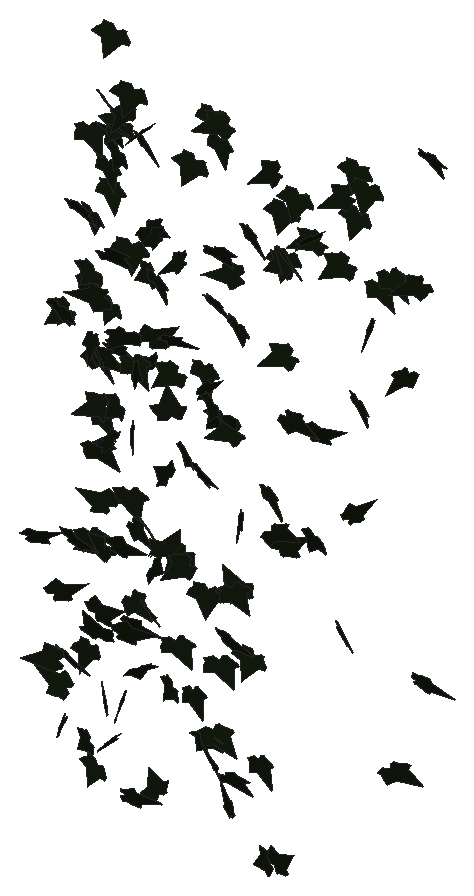
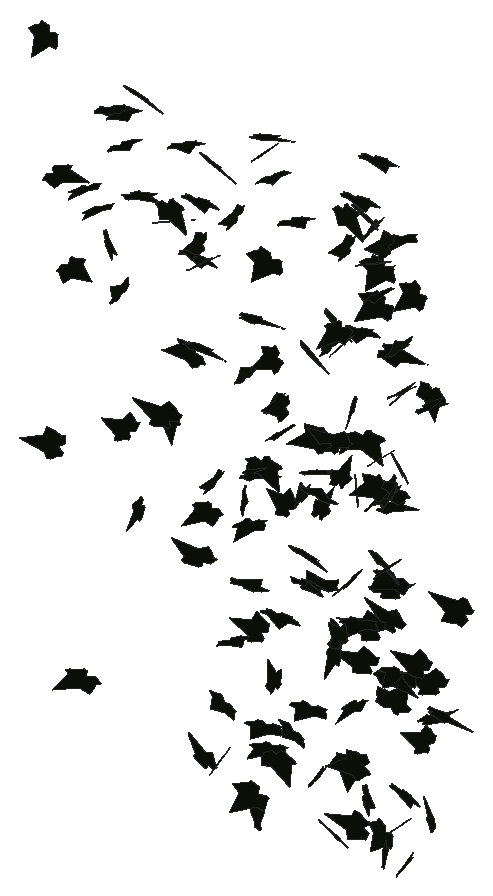
# SketchUp Ruby script. Lengths in inches.
U = 1.inch
M = Sketchup.active_model
def pt(a) = Geom::Point3d.new(a.map { |v| v * U })
def face(e, loops, mat)
  f = e.add_face(loops[0].map { |a| pt(a) })
  loops[1..].each { |l| e.add_face(l.map { |a| pt(a) }).erase! }
  f.material = f.back_material = mat if mat
  f
end
# faces: each face lists its corners as indices into pts; further lists are holes
def faces(e, pts, list, mat = nil) = list.each { |f| face(e, (f[0].is_a?(Array) ? f : [f]).map { |l| l.map { |i| pts[i] } }, mat) }
# xy, xz, yz: faces in a plane at the given z, y or x. An outline is a flat list of corners, or four numbers for a rectangle; further outlines are holes
def ring(l) = l.size == 4 ? [[l[0], l[1]], [l[2], l[1]], [l[2], l[3]], [l[0], l[3]]] : l.each_slice(2).to_a
def flat(e, list, mat, &to3) = list.each { |f| face(e, (f[0].is_a?(Array) ? f : [f]).map { |l| ring(l).map { |u, v| to3.(u, v) } }, mat) }
def xy(e, z, list, mat = nil) = flat(e, list, mat) { |x, y| [x, y, z] }
def xz(e, y, list, mat = nil) = flat(e, list, mat) { |x, z| [x, y, z] }
def yz(e, x, list, mat = nil) = flat(e, list, mat) { |y, z| [x, y, z] }
def lines(e, pts, list) = list.each { |a, b| e.add_line(pt(pts[a]), pt(pts[b])) }
# prism: a flat outline (further loops are holes) pulled along v
def prism(e, loops, v, mat = nil)
  f = face(e, loops, mat); d = Geom::Vector3d.new(v.map { |x| x * U })
  f.pushpull(f.normal.samedirection?(d) ? d.length : -d.length)
end
def box(e, o, s, mat = nil) = prism(e, [[o, [o[0] + s[0], o[1], o[2]], [o[0] + s[0], o[1] + s[1], o[2]], [o[0], o[1] + s[1], o[2]]]], [0, 0, s[2]], mat)
def at(x, y, z, deg = 0) = Geom::Transformation.translation(pt([x, y, z])) * Geom::Transformation.rotation(ORIGIN, Z_AXIS, deg.degrees)
def axes(o, x, y, z) = Geom::Transformation.new([*x, 0, *y, 0, *z, 0, *pt(o).to_a, 1])
def part(name) = M.definitions.add(name)
# library, detail: a bought-in or finely detailed component or shape, given as its bounding box
def library(name, o, s) = part(name).tap { |d| box(d.entities, o, s) }
def detail(e, o, s) = box(e.add_group.entities, o, s)
def put(e, d, t, mat = nil) = e.add_instance(d, t).tap { |i| i.material = mat if mat }
def group(e, t, mat = nil) = e.add_group.tap { |g| g.transformation = t; g.material = mat if mat }.entities
root = M.entities
M.materials.add("1026 AP 7946 SUNNY SIDE UP").color = [254, 231, 186]
M.materials.add("efeu1").color = [18, 25, 13]
c1 = part("ivyleaf_9")
p = [[1.54,2.16,1.25],[1.36,2.04,1.19],[-0.21,0.99,0.68],[-0.71,1.11,0.82],[-0.85,0.86,0.67],[-0.8,0.17,0.21],
  [-0.9,-0.01,0.1],[-0.67,-0.16,-0.02],[-0.08,-0.08,-0.05],[-0.03,-0.6,-0.4],[0.65,-0.88,-0.66],[0.83,-0.6,-0.49],
  [1.29,-0.42,-0.43],[1.8125,-0.07,-0.26],[1.21,0.44,0.15]]
faces(c1.entities,p,[[0,1,2,3,4,5,6,7,8,9,10,11,12,13,14]],"efeu1")
put(root,c1,axes([176.66,210.71,296.68],[-0.62079,-0.06048,-0.24475],[0.37867,-0.01488,-0.40905],[0.06932,-0.46036,0.04263]),"1026 AP 7946 SUNNY SIDE UP")
put(root,c1,axes([176.78,208.77,316.86],[-0.34325,-0.29743,0.3129],[-0.25777,-0.25818,-0.38123],[0.61879,-0.27253,0.01475]),"1026 AP 7946 SUNNY SIDE UP")
put(root,c1,axes([176.43,211.22,321.1875],[-0.03798,-0.39245,0.26497],[0.11301,-0.2598,-0.3995],[0.73105,0.01977,0.07552]),"1026 AP 7946 SUNNY SIDE UP")
put(root,c1,axes([176.24,206.52,304.73],[0.51781,0.27509,-0.19939],[0.19907,0.15193,0.44169],[0.49153,-0.35133,0.03117]),"1026 AP 7946 SUNNY SIDE UP")
put(root,c1,axes([176.3,212.23,327.35],[0.50505,-0.33544,0.1326],[0.09947,-0.11973,-0.47773],[0.55722,0.32541,-0.0349]),"1026 AP 7946 SUNNY SIDE UP")
put(root,c1,axes([176.2,209.78,303.16],[0.29433,-0.17747,0.41107],[0.49315,-0.24903,-0.26646],[0.47991,0.36475,0.02171]),"1026 AP 7946 SUNNY SIDE UP")
put(root,c1,axes([176.51,211.81,309.54],[0.19314,-0.42841,-0.13884],[-0.02652,0.13271,-0.45791],[0.70454,0.12244,0.02083]),"1026 AP 7946 SUNNY SIDE UP")
put(root,c1,axes([176.93,208.05,317.375],[0.51444,0.00554,-0.35204],[-0.52619,-0.09112,-0.33208],[-0.10941,0.46425,-0.05816]),"1026 AP 7946 SUNNY SIDE UP")
put(root,c1,axes([176.74,212.39,315.56],[-0.17337,-0.35996,0.21476],[-0.02551,-0.21388,-0.38676],[0.65519,-0.10358,0.04177]),"1026 AP 7946 SUNNY SIDE UP")
put(root,c1,axes([176.875,211.03,313.57],[0.46463,-0.22327,-0.28441],[-0.39252,0.12246,-0.37832],[0.39483,0.38449,-0.04142]),"1026 AP 7946 SUNNY SIDE UP")
put(root,c1,axes([176.66,210.78,303.15],[-0.25406,-0.21807,-0.38632],[0.38165,0.28462,-0.27751],[0.56331,-0.29119,0.01378]),"1026 AP 7946 SUNNY SIDE UP")
put(root,c1,axes([176.79,211.96,325.92],[0.69115,0.13249,-0.08852],[-0.10161,-0.08337,-0.46936],[-0.22728,0.44019,-0.05935]),"1026 AP 7946 SUNNY SIDE UP")
put(root,c1,axes([176.97,210.64,318.3],[-0.35108,-0.28922,0.29586],[-0.041,-0.31837,-0.35105],[0.64141,-0.17866,0.1395]),"1026 AP 7946 SUNNY SIDE UP")
put(root,c1,axes([177.51,210.74,302.82],[0.026,-0.01704,-0.47108],[-0.57664,-0.27401,-0.00474],[-0.43009,0.36634,-0.02212]),"1026 AP 7946 SUNNY SIDE UP")
put(root,c1,axes([176.93,210.64,314.49],[-0.43021,0.02432,-0.39229],[0.56896,-0.1327,-0.27724],[-0.19109,-0.44984,0.05771]),"1026 AP 7946 SUNNY SIDE UP")
put(root,c1,axes([176.74,211.29,313.15],[0.35166,-0.39736,-0.04156],[-0.03147,0.03244,-0.46955],[0.62688,0.22453,-0.00026]),"1026 AP 7946 SUNNY SIDE UP")
put(root,c1,axes([177.28,211.3,293.05],[-0.00904,-0.18472,0.40636],[0.04608,0.39447,0.19255],[-0.68482,0.02898,0.00759]),"1026 AP 7946 SUNNY SIDE UP")
put(root,c1,axes([176.75,211.08,313.36],[0.0638,-0.0925,-0.47457],[0.3914,0.39579,-0.05704],[0.62566,-0.23817,0.08408]),"1026 AP 7946 SUNNY SIDE UP")
put(root,c1,axes([176.99,209.97,318.18],[0.28007,-0.41904,-0.12282],[-0.08877,0.10292,-0.46833],[0.67825,0.1865,-0.01058]),"1026 AP 7946 SUNNY SIDE UP")
put(root,c1,axes([177.09,207.82,293.42],[0.05621,0.26537,0.34627],[-0.06691,-0.3319,0.27391],[0.66819,-0.05556,-0.0017]),"1026 AP 7946 SUNNY SIDE UP")
put(root,c1,axes([177.04,210.25,326.7],[-0.08134,-0.41139,-0.23378],[0.09107,0.21861,-0.42499],[0.73134,-0.07297,0.02692]),"1026 AP 7946 SUNNY SIDE UP")
put(root,c1,axes([177.34,212.43,326.11],[-0.48774,-0.32332,0.1613],[0.00489,-0.21148,-0.43966],[0.56611,-0.27674,0.14276]),"1026 AP 7946 SUNNY SIDE UP")
put(root,c1,axes([177.25,209.93,291.82],[-0.16792,-0.16998,0.40395],[-0.12439,-0.39031,-0.1983],[0.66179,-0.11649,0.06522]),"1026 AP 7946 SUNNY SIDE UP")
put(root,c1,axes([176.87,207.82,301.1],[0.04149,0.01406,0.48813],[0.72236,0.11593,-0.02923],[-0.18327,0.4601,-0.00469]),"1026 AP 7946 SUNNY SIDE UP")
put(root,c1,axes([177.41,211.85,331.65],[-0.62146,-0.24372,-0.12609],[0.20704,0.01545,-0.475],[0.37444,-0.41305,0.05337]),"1026 AP 7946 SUNNY SIDE UP")
put(root,c1,axes([177.02,210.83,308.28],[-0.16999,-0.13214,-0.44594],[0.48022,0.3061,-0.17335],[0.52367,-0.3236,0.01421]),"1026 AP 7946 SUNNY SIDE UP")
put(root,c1,axes([177.11,208.91,322.98],[0.73184,-0.07926,-0.02833],[-0.05326,-0.0385,-0.48454],[0.12044,0.46462,-0.04216]),"1026 AP 7946 SUNNY SIDE UP")
put(root,c1,axes([178.16,206.2,298.44],[-0.59478,0.131,0.26622],[-0.40522,0.03937,-0.41013],[-0.20586,-0.45599,0.03816]),"1026 AP 7946 SUNNY SIDE UP")
put(root,c1,axes([177.15,211.8,313.65],[0.64815,-0.02989,0.13586],[0.1987,-0.06695,-0.42238],[0.07641,0.42763,-0.05406]),"1026 AP 7946 SUNNY SIDE UP")
put(root,c1,axes([178.14,210.6875,308.99],[-0.41016,0.35242,0.08873],[-0.11772,0.049,-0.45031],[-0.55742,-0.26966,0.02981]),"1026 AP 7946 SUNNY SIDE UP")
put(root,c1,axes([178.24,209.89,311.34],[-0.50112,-0.17584,0.30822],[-0.37278,-0.18818,-0.37394],[0.40035,-0.39531,0.03761]),"1026 AP 7946 SUNNY SIDE UP")
put(root,c1,axes([177.4,207.83,297.77],[0.37377,-0.27426,0.31055],[0.33544,-0.21572,-0.37483],[0.54814,0.31903,0.01762]),"1026 AP 7946 SUNNY SIDE UP")
put(root,c1,axes([177.74,210.85,324.68],[0.06205,-0.47249,0.0648],[0.0049,-0.06555,-0.48883],[0.75005,0.03952,-0.00217]),"1026 AP 7946 SUNNY SIDE UP")
put(root,c1,axes([178.03,210.77,323.5],[-0.05815,-0.46712,-0.02027],[-0.00965,0.01756,-0.48257],[0.73493,-0.03673,-0.00794]),"1026 AP 7946 SUNNY SIDE UP")
put(root,c1,axes([178.92,209.31,306.2],[-0.07979,0.08198,0.45897],[-0.70589,-0.06557,-0.04067],[0.0897,-0.44311,0.0882]),"1026 AP 7946 SUNNY SIDE UP")
put(root,c1,axes([178.73,211.21,327.9],[-0.63622,-0.01116,-0.25311],[0.36454,-0.17488,-0.38627],[-0.1288,-0.43985,0.15701]),"1026 AP 7946 SUNNY SIDE UP")
put(root,c1,axes([178.91,210.78,315.37],[0.21758,0.24064,-0.39838],[-0.25627,-0.35276,-0.28729],[-0.6707,0.21285,-0.01946]),"1026 AP 7946 SUNNY SIDE UP")
put(root,c1,axes([178.14,211.87,298.05],[0.56527,0.0027,0.27538],[0.41884,-0.04098,-0.36889],[0.03506,0.44609,-0.03292]),"1026 AP 7946 SUNNY SIDE UP")
put(root,c1,axes([178.49,211.61,305.74],[-0.25565,-0.34144,-0.2904],[0.22633,0.24104,-0.38757],[0.65634,-0.21612,0.02053]),"1026 AP 7946 SUNNY SIDE UP")
put(root,c1,axes([179.12,205.67,297.49],[-0.36991,-0.40501,-0.08415],[-0.06792,-0.06671,0.48211],[-0.6454,0.23916,-0.0025]),"1026 AP 7946 SUNNY SIDE UP")
put(root,c1,axes([178.79,211.52,328.87],[-0.6171,-0.2234,-0.1631],[0.26314,0.02054,-0.46078],[0.33931,-0.42221,0.06072]),"1026 AP 7946 SUNNY SIDE UP")
put(root,c1,axes([178.83,210.3125,311.43],[-0.17688,-0.26822,0.33727],[-0.17166,-0.31053,-0.30116],[0.64489,-0.15622,0.01234]),"1026 AP 7946 SUNNY SIDE UP")
put(root,c1,axes([179.44,208.25,318.75],[-0.25175,-0.10611,-0.45155],[-0.45796,-0.32996,0.19022],[-0.54021,0.32917,0.04918]),"1026 AP 7946 SUNNY SIDE UP")
put(root,c1,axes([179.28,208.19,299.375],[0.44654,-0.11305,0.36897],[-0.48891,0.18251,0.31384],[-0.33295,-0.41961,0.034]),"1026 AP 7946 SUNNY SIDE UP")
put(root,c1,axes([179.13,208.9,292.76],[0.19534,0.3464,0.30483],[0.15127,0.27775,-0.37748],[-0.69813,0.1571,0.0035]),"1026 AP 7946 SUNNY SIDE UP")
put(root,c1,axes([179.14,209.95,326.17],[-0.08365,-0.33255,0.34235],[-0.02163,-0.33509,-0.34771],[0.74102,-0.04732,0.02849]),"1026 AP 7946 SUNNY SIDE UP")
put(root,c1,axes([179.04,211.83,326.15],[0.4373,-0.3765,0.06903],[0.02872,-0.07231,-0.48177],[0.60122,0.2773,-0.02719]),"1026 AP 7946 SUNNY SIDE UP")
put(root,c1,axes([179.54,211.82,313.14],[0.14933,0.15978,0.43145],[-0.45831,-0.30202,0.18543],[0.53373,-0.30405,0.03852]),"1026 AP 7946 SUNNY SIDE UP")
put(root,c1,axes([179.44,210.01,295.16],[-0.30628,0.09838,-0.43053],[0.51909,-0.26004,-0.2228],[-0.43296,-0.38137,0.03744]),"1026 AP 7946 SUNNY SIDE UP")
put(root,c1,axes([179.53,207.67,292.25],[-0.17445,-0.38785,0.25209],[-0.06195,-0.24504,-0.41621],[0.72029,-0.11501,0.02526]),"1026 AP 7946 SUNNY SIDE UP")
put(root,c1,axes([179.47,210.66,300.46],[0.17201,-0.28495,-0.36742],[-0.12935,0.34676,-0.31079],[0.70404,0.13332,0.03266]),"1026 AP 7946 SUNNY SIDE UP")
put(root,c1,axes([179.625,210.4,320.82],[-0.44277,-0.3393,-0.18952],[0.25029,0.10277,-0.4504],[0.55129,-0.31917,0.05228]),"1026 AP 7946 SUNNY SIDE UP")
put(root,c1,axes([180.04,210.82,327.35],[-0.24911,0.41378,-0.18412],[0.04346,-0.18265,-0.45597],[-0.70887,-0.15661,0.03675]),"1026 AP 7946 SUNNY SIDE UP")
put(root,c1,axes([179.7,211.57,321.36],[-0.00071,-0.03977,-0.49257],[-0.16392,0.46649,-0.03716],[0.73603,0.10385,-0.00875]),"1026 AP 7946 SUNNY SIDE UP")
put(root,c1,axes([179.33,209.39,303.98],[0.37335,-0.0321,0.42007],[0.60906,-0.13445,-0.24395],[0.20747,0.45246,-0.03979]),"1026 AP 7946 SUNNY SIDE UP")
put(root,c1,axes([179.7,208.37,321.3],[0.69971,0.14828,0.07105],[0.12532,-0.02483,-0.48079],[-0.2239,0.44949,-0.04708]),"1026 AP 7946 SUNNY SIDE UP")
put(root,c1,axes([180.17,210.26,296.86],[0.22314,0.44715,-0.02356],[0.0083,-0.02832,-0.48325],[-0.70418,0.14136,-0.01316]),"1026 AP 7946 SUNNY SIDE UP")
put(root,c1,axes([179.79,211.44,304.21],[0.14554,-0.27258,0.38444],[0.19568,-0.35346,-0.29862],[0.70184,0.15507,0.00354]),"1026 AP 7946 SUNNY SIDE UP")
put(root,c1,axes([179.83,211.64,314.9],[-0.14628,0.01606,0.47274],[0.71854,0.04803,0.09401],[-0.06907,0.46566,-0.02324]),"1026 AP 7946 SUNNY SIDE UP")
put(root,c1,axes([180.01,210.07,314.51],[0.02377,-0.42849,-0.2288],[0.05332,0.22017,-0.43876],[0.75525,-0.00206,0.03818]),"1026 AP 7946 SUNNY SIDE UP")
put(root,c1,axes([180.81,211.02,321.47],[-0.54211,0.28564,-0.0632],[0.05585,-0.05573,-0.4611],[-0.45652,-0.34601,0.01864]),"1026 AP 7946 SUNNY SIDE UP")
put(root,c1,axes([180.68,210.66,319.41],[-0.24334,-0.15146,0.40186],[-0.21243,-0.37648,-0.20756],[0.62408,-0.18721,0.08604]),"1026 AP 7946 SUNNY SIDE UP")
put(root,c1,axes([180.86,210.5625,302.8125],[0.03128,-0.0739,-0.48345],[-0.46249,0.3664,-0.07021],[0.58578,0.29323,-0.02962]),"1026 AP 7946 SUNNY SIDE UP")
put(root,c1,axes([181.05,212.13,313.27],[-0.55807,-0.22618,0.17291],[-0.11038,-0.19245,-0.41802],[0.43015,-0.34283,0.11707]),"1026 AP 7946 SUNNY SIDE UP")
put(root,c1,axes([180.58,209.24,311.17],[-0.05449,-0.07884,-0.48389],[0.67086,-0.21348,0.00325],[-0.3313,-0.41932,0.08616]),"1026 AP 7946 SUNNY SIDE UP")
put(root,c1,axes([180.57,211.91,315.13],[0.57376,0.06185,0.24587],[0.35842,0.07618,-0.37948],[-0.14634,0.42911,0.03457]),"1026 AP 7946 SUNNY SIDE UP")
put(root,c1,axes([181.5,212.01,319.88],[-0.58098,0.25479,-0.07206],[0.0663,-0.06436,-0.4618],[-0.41075,-0.37078,0.02738]),"1026 AP 7946 SUNNY SIDE UP")
put(root,c1,axes([181.45,211.26,311.45],[-0.73186,0.05825,0.03177],[0.05583,0.03906,0.48142],[0.08703,0.4648,-0.04166]),"1026 AP 7946 SUNNY SIDE UP")
put(root,c1,axes([181.04,208.84,306.01],[0.40449,-0.34384,-0.21981],[-0.13872,0.19675,-0.43907],[0.61933,0.26863,0.04522]),"1026 AP 7946 SUNNY SIDE UP")
put(root,c1,axes([181.5,208.28,315.26],[0.20364,-0.11127,-0.4361],[-0.50341,0.27599,-0.17429],[0.4679,0.34535,0.00229]),"1026 AP 7946 SUNNY SIDE UP")
put(root,c1,axes([181.1,210.52,319.42],[0.16858,-0.41869,0.1819],[0.08894,-0.17016,-0.44608],[0.71041,0.12066,0.01269]),"1026 AP 7946 SUNNY SIDE UP")
put(root,c1,axes([180.95,205.97,302.24],[0.00357,0.05292,0.49089],[0.57467,-0.30814,0.03168],[0.48719,0.36308,-0.04097]),"1026 AP 7946 SUNNY SIDE UP")
put(root,c1,axes([181.49,211.27,295.84],[-0.11596,-0.26341,0.36242],[-0.07162,-0.35173,-0.28202],[0.68922,-0.08087,0.03167]),"1026 AP 7946 SUNNY SIDE UP")
put(root,c1,axes([181.33,207.44,300.55],[0.22029,0.02305,0.45644],[0.68932,-0.07771,-0.13913],[0.10586,0.45801,-0.04381]),"1026 AP 7946 SUNNY SIDE UP")
put(root,c1,axes([182.76,208.57,291.45],[-0.62875,0.12343,-0.24255],[-0.33573,0.10633,0.43035],[0.25065,0.45205,-0.03201]),"1026 AP 7946 SUNNY SIDE UP")
put(root,c1,axes([181.76,207.38,291.47],[0.39275,0.13523,-0.36289],[0.4435,0.21506,0.29171],[0.39578,-0.37518,0.03322]),"1026 AP 7946 SUNNY SIDE UP")
put(root,c1,axes([182.29,208.29,301.85],[0.49785,-0.15166,-0.27806],[0.40883,-0.07707,0.35951],[-0.26211,-0.40828,0.03262]),"1026 AP 7946 SUNNY SIDE UP")
put(root,c1,axes([182.73,211.53,326.21],[-0.42435,-0.38509,0.0734],[-0.02635,-0.07774,-0.48387],[0.61586,-0.26867,0.02987]),"1026 AP 7946 SUNNY SIDE UP")
put(root,c1,axes([182.45,210.43,299.15],[-0.23605,-0.26406,-0.35182],[0.30747,0.27898,-0.31052],[0.60308,-0.24559,0.0206]),"1026 AP 7946 SUNNY SIDE UP")
put(root,c1,axes([182.79,209.27,309.18],[0.09389,0.10559,0.46261],[-0.43493,-0.35342,0.1216],[0.57934,-0.28243,0.01632]),"1026 AP 7946 SUNNY SIDE UP")
put(root,c1,axes([182.89,209.04,304.89],[-0.46773,-0.03384,0.38614],[0.56888,0.10677,0.30618],[-0.16409,0.4666,-0.03917]),"1026 AP 7946 SUNNY SIDE UP")
put(root,c1,axes([183.2,210.28,310.18],[-0.0419,-0.23912,0.39293],[0.04086,-0.38362,-0.24727],[0.70849,0.00798,0.0375]),"1026 AP 7946 SUNNY SIDE UP")
put(root,c1,axes([183.29,212.37,328.79],[-0.18827,-0.46383,0.00713],[0.00915,-0.01137,-0.49348],[0.72942,-0.11957,0.00803]),"1026 AP 7946 SUNNY SIDE UP")
put(root,c1,axes([183.24,211.71,314.53],[0.00685,-0.48184,-0.00698],[-0.00295,0.00402,-0.49638],[0.75767,0.00437,-0.00187]),"1026 AP 7946 SUNNY SIDE UP")
put(root,c1,axes([183.76,209.42,305.14],[-0.67396,-0.14127,-0.04458],[0.08477,-0.02853,-0.4629],[0.21591,-0.42977,0.04258]),"1026 AP 7946 SUNNY SIDE UP")
put(root,c1,axes([183.49,211.8,318.51],[0.66712,-0.14494,0.01664],[0.00416,-0.04454,-0.46018],[0.22942,0.42227,-0.04004]),"1026 AP 7946 SUNNY SIDE UP")
put(root,c1,axes([184.53,211.52,312.3],[0.28012,0.17456,-0.38597],[-0.42818,-0.25879,-0.25844],[-0.49081,0.32539,0.00517]),"1026 AP 7946 SUNNY SIDE UP")
put(root,c1,axes([183.98,209.87,297.07],[-0.29724,-0.10648,-0.41498],[0.63997,0.04439,-0.20891],[0.13582,-0.44219,0.07619]),"1026 AP 7946 SUNNY SIDE UP")
put(root,c1,axes([184.22,211.68,298.09],[-0.24036,-0.28398,-0.33709],[0.28994,0.26946,-0.32972],[0.61436,-0.23827,0.02373]),"1026 AP 7946 SUNNY SIDE UP")
put(root,c1,axes([184.01,210.23,309.46],[0.21541,-0.22211,0.40828],[0.3338,-0.33617,-0.27079],[0.63353,0.25264,0.00385]),"1026 AP 7946 SUNNY SIDE UP")
put(root,c1,axes([185.06,212.01,320.27],[-0.55727,0.04516,0.28135],[-0.43461,-0.07298,-0.35784],[0.01484,-0.44127,0.0853]),"1026 AP 7946 SUNNY SIDE UP")
put(root,c1,axes([184.65,209.68,314.46],[0.10681,0.14596,0.43673],[0.41377,0.33314,-0.15997],[-0.56927,0.26953,-0.03433]),"1026 AP 7946 SUNNY SIDE UP")
put(root,c1,axes([185.1875,211.75,311.53],[-0.45897,-0.16522,0.31536],[-0.39339,-0.1797,-0.34566],[0.38191,-0.38366,0.02294]),"1026 AP 7946 SUNNY SIDE UP")
put(root,c1,axes([185.19,207.87,305.625],[-0.73678,0.02805,-0.00923],[0.00998,-0.04591,-0.48158],[-0.04529,-0.46641,0.04408]),"1026 AP 7946 SUNNY SIDE UP")
put(root,c1,axes([185.31,210.74,329.56],[-0.62592,-0.08814,0.25039],[-0.30359,-0.1967,-0.39958],[0.27148,-0.42318,0.13046]),"1026 AP 7946 SUNNY SIDE UP")
put(root,c1,axes([184.875,209.91,303.15],[-0.52722,-0.25151,-0.23447],[0.33656,0.08882,-0.42813],[0.41182,-0.39457,0.04972]),"1026 AP 7946 SUNNY SIDE UP")
put(root,c1,axes([185.26,209.45,295.05],[0.36462,0.16127,-0.37271],[-0.47046,-0.20502,-0.29217],[-0.41015,0.37853,0.0038]),"1026 AP 7946 SUNNY SIDE UP")
put(root,c1,axes([184.875,212.34,317.25],[0.02203,-0.36907,0.2631],[0.10978,-0.25271,-0.37855],[0.69903,0.05132,0.05116]),"1026 AP 7946 SUNNY SIDE UP")
put(root,c1,axes([185.13,210.16,322.62],[0.67476,0.15067,-0.05148],[-0.05242,-0.05777,-0.46676],[-0.24447,0.42824,-0.04199]),"1026 AP 7946 SUNNY SIDE UP")
put(root,c1,axes([185.13,210.56,328.6875],[0.03878,-0.47064,0.03838],[-0.00074,-0.04,-0.48575],[0.7427,0.02454,-0.00249]),"1026 AP 7946 SUNNY SIDE UP")
put(root,c1,axes([185.46,209.56,314.15],[-0.06869,-0.30738,0.33931],[0.00879,-0.333,-0.31965],[0.71034,-0.0256,0.03676]),"1026 AP 7946 SUNNY SIDE UP")
put(root,c1,axes([185.58,209.55,295.51],[-0.01847,-0.32919,-0.36315],[0.23502,0.33088,-0.32324],[0.7188,-0.11664,0.09636]),"1026 AP 7946 SUNNY SIDE UP")
put(root,c1,axes([186.59,209.52,291.26],[0.04363,-0.12771,0.47782],[-0.12332,0.4579,0.13719],[-0.74744,-0.08301,0.00526]),"1026 AP 7946 SUNNY SIDE UP")
put(root,c1,axes([186.09,209.98,292.89],[0.73144,0.11421,0.04205],[0.078,-0.03433,-0.49147],[-0.17365,0.46564,-0.04364]),"1026 AP 7946 SUNNY SIDE UP")
put(root,c1,axes([187.17,209.65,303.82],[-0.72138,-0.14531,-0.01368],[-0.03302,0.02514,0.49493],[-0.22694,0.45826,-0.02853]),"1026 AP 7946 SUNNY SIDE UP")
put(root,c1,axes([186.53,209.18,301.29],[0.38693,-0.19155,0.37105],[0.42512,-0.2401,-0.32228],[0.48236,0.36526,-0.01361]),"1026 AP 7946 SUNNY SIDE UP")
put(root,c1,axes([187.07,210.33,324.36],[0.39995,-0.40882,0.03101],[-0.00648,-0.0407,-0.4956],[0.64482,0.25316,-0.02421]),"1026 AP 7946 SUNNY SIDE UP")
put(root,c1,axes([187.34,209.47,308.43],[-0.08134,0.00826,-0.47272],[0.57298,-0.28006,-0.04915],[-0.43882,-0.36721,0.02345]),"1026 AP 7946 SUNNY SIDE UP")
put(root,c1,axes([188.125,211.23,327.6],[-0.69121,0.17546,0.01833],[-0.04003,-0.01856,-0.48694],[-0.27425,-0.43952,0.02489]),"1026 AP 7946 SUNNY SIDE UP")
put(root,c1,axes([187.93,209.71,300.56],[-0.36561,-0.40988,0.08946],[-0.03552,-0.08957,-0.48536],[0.65862,-0.23236,0.02349]),"1026 AP 7946 SUNNY SIDE UP")
put(root,c1,axes([188.1875,212.05,322.02],[-0.39405,-0.16945,0.36703],[-0.23677,-0.35017,-0.28199],[0.57485,-0.26039,0.13544]),"1026 AP 7946 SUNNY SIDE UP")
put(root,c1,axes([188.26,211.99,322.5625],[-0.56698,-0.20469,-0.21267],[0.34974,0.01475,-0.41757],[0.29232,-0.41466,0.08711]),"1026 AP 7946 SUNNY SIDE UP")
put(root,c1,axes([188.75,211.51,317.23],[-0.69536,-0.03655,0.12835],[-0.18697,-0.06539,-0.4542],[0.08276,-0.45482,0.05226]),"1026 AP 7946 SUNNY SIDE UP")
put(root,c1,axes([188.42,211.68,325.46],[-0.58566,-0.21648,-0.17335],[0.27708,0.02579,-0.43907],[0.32875,-0.40739,0.06125]),"1026 AP 7946 SUNNY SIDE UP")
put(root,c1,axes([188.1,210.67,309.62],[0.31683,-0.42813,0.05224],[0.0013,-0.05827,-0.48718],[0.67835,0.20007,-0.02347]),"1026 AP 7946 SUNNY SIDE UP")
put(root,c1,axes([188.04,211.8,305.83],[-0.16048,0.04371,0.46335],[0.6962,-0.08124,0.11122],[0.14012,0.45374,-0.02195]),"1026 AP 7946 SUNNY SIDE UP")
put(root,c1,axes([188.29,205.9,296.29],[-0.02797,-0.11253,0.47095],[0.1643,-0.44766,-0.1118],[0.72282,0.0974,0.04364]),"1026 AP 7946 SUNNY SIDE UP")
put(root,c1,axes([188.24,211.58,322.95],[0.53756,-0.33436,0.02375],[-0.00866,-0.04123,-0.49169],[0.52714,0.3403,-0.0323]),"1026 AP 7946 SUNNY SIDE UP")
put(root,c1,axes([188.58,207.28,305.71],[-0.02478,-0.34867,-0.33704],[0.02297,0.32486,-0.35766],[0.74933,-0.02149,-0.00018]),"1026 AP 7946 SUNNY SIDE UP")
put(root,c1,axes([188.72,210.3125,307.72],[0.01251,-0.02103,-0.48526],[-0.02334,0.47074,-0.01916],[0.74085,0.01518,0.00759]),"1026 AP 7946 SUNNY SIDE UP")
put(root,c1,axes([190,212.23,323.89],[-0.60392,-0.11939,0.25997],[-0.21428,-0.29548,-0.35847],[0.38421,-0.35246,0.2087]),"1026 AP 7946 SUNNY SIDE UP")
put(root,c1,axes([190.16,211.63,324.45],[-0.14665,0.40297,-0.21322],[0.00082,-0.21353,-0.42511],[-0.71398,-0.08302,0.04331]),"1026 AP 7946 SUNNY SIDE UP")
put(root,c1,axes([189.64,208.07,295.86],[-0.27066,-0.07351,-0.43991],[0.66245,0.07706,-0.18836],[0.15642,-0.45351,0.0365]),"1026 AP 7946 SUNNY SIDE UP")
put(root,c1,axes([190.21,210.49,327.32],[-0.36984,-0.40582,-0.0097],[0.04401,-0.00801,-0.48238],[0.63669,-0.23518,0.02771]),"1026 AP 7946 SUNNY SIDE UP")
put(root,c1,axes([189.95,211.97,312.95],[0.08924,-0.04749,0.48082],[0.72051,-0.09646,-0.06804],[0.16015,0.46044,0.03818]),"1026 AP 7946 SUNNY SIDE UP")
put(root,c1,axes([190.5,209.33,315.26],[0.10219,-0.06914,-0.46735],[0.6199,0.24216,0.0216],[0.36809,-0.38862,0.09338]),"1026 AP 7946 SUNNY SIDE UP")
put(root,c1,axes([191.16,206.86,291.16],[-0.17991,-0.0909,0.45659],[-0.22604,-0.42671,-0.13074],[0.67538,-0.16703,0.07787]),"1026 AP 7946 SUNNY SIDE UP")
put(root,c1,axes([191.7,206.8,291.26],[-0.15719,0.14717,0.44706],[0.36481,-0.36578,0.18107],[0.61991,0.25258,0.00681]),"1026 AP 7946 SUNNY SIDE UP")
put(root,c1,axes([192.66,211.18,323.97],[-0.59984,-0.2182,0.17186],[-0.18777,-0.12769,-0.45077],[0.39026,-0.39682,0.04728]),"1026 AP 7946 SUNNY SIDE UP")
put(root,c1,axes([192.57,212.31,328.95],[-0.30969,-0.42261,0.04574],[-0.00571,-0.0499,-0.48028],[0.66855,-0.19619,0.01709]),"1026 AP 7946 SUNNY SIDE UP")
put(root,c1,axes([193.08,211.64,326.78],[-0.2803,-0.42513,0.09146],[-0.04208,-0.08765,-0.47533],[0.68239,-0.18003,0.00825]),"1026 AP 7946 SUNNY SIDE UP")
put(root,c1,axes([193.36,207.72,310.17],[0.45387,-0.0079,-0.37903],[-0.57573,-0.05253,-0.29511],[-0.05737,0.46464,-0.03706]),"1026 AP 7946 SUNNY SIDE UP")
put(root,c1,axes([193.75,209.95,328.77],[-0.72139,0.12611,0.02921],[-0.06377,-0.04391,-0.48737],[-0.19273,-0.45751,0.05193]),"1026 AP 7946 SUNNY SIDE UP")
put(root,c1,axes([193.73,211.61,328.55],[-0.38438,-0.40223,-0.04611],[0.0595,0.02667,-0.48437],[0.63319,-0.24668,0.01752]),"1026 AP 7946 SUNNY SIDE UP")
put(root,c1,axes([193.71,210.28,310.27],[0.01239,-0.04346,0.49478],[0.62073,0.27689,0.02075],[-0.43619,0.3928,0.04358]),"1026 AP 7946 SUNNY SIDE UP")
put(root,c1,axes([194.2,211.33,321.02],[-0.37025,0.12215,-0.40266],[0.50756,-0.22337,-0.27307],[-0.39792,-0.39858,0.02635]),"1026 AP 7946 SUNNY SIDE UP")
put(root,c1,axes([194.1875,211.86,323.04],[0.07792,-0.4209,-0.21],[0.06755,0.20584,-0.43096],[0.73061,0.02586,0.06224]),"1026 AP 7946 SUNNY SIDE UP")
put(root,c1,axes([194.48,208.39,304.99],[0.53621,-0.22338,-0.25877],[-0.35727,0.10807,-0.41827],[0.3875,0.40874,-0.02756]),"1026 AP 7946 SUNNY SIDE UP")
put(root,c1,axes([194.53,209.86,317.33],[0.18739,-0.39217,0.24968],[0.07614,-0.24061,-0.42315],[0.72276,0.12703,-0.02016]),"1026 AP 7946 SUNNY SIDE UP")
put(root,c1,axes([194.97,211.88,323.89],[0.08324,-0.41166,-0.23307],[0.07827,0.22899,-0.42026],[0.73267,0.02231,0.07138]),"1026 AP 7946 SUNNY SIDE UP")
put(root,c1,axes([195.83,210.94,296.33],[0.00402,-0.05546,-0.49237],[0.20514,0.45979,-0.05159],[0.7277,-0.12931,0.01726]),"1026 AP 7946 SUNNY SIDE UP")
put(root,c1,axes([196.39,211.42,318.89],[-0.0412,0.14248,-0.4704],[0.14736,-0.44774,-0.15182],[-0.73879,-0.09725,-0.00405]),"1026 AP 7946 SUNNY SIDE UP")
put(root,c1,axes([196.875,211.89,324.01],[-0.05605,-0.0617,-0.48715],[-0.06389,-0.47172,0.06385],[-0.74657,0.045,0.03111]),"1026 AP 7946 SUNNY SIDE UP")
put(root,c1,axes([197.33,211.89,331.52],[0.71627,-0.02114,-0.15009],[-0.23072,-0.03178,-0.46844],[0.01636,0.47716,-0.03504]),"1026 AP 7946 SUNNY SIDE UP")
put(root,c1,axes([201.14,206.47,305.15],[0.52035,-0.11779,0.33882],[0.47216,-0.13741,-0.36203],[0.28267,0.44636,-0.019]),"1026 AP 7946 SUNNY SIDE UP")
